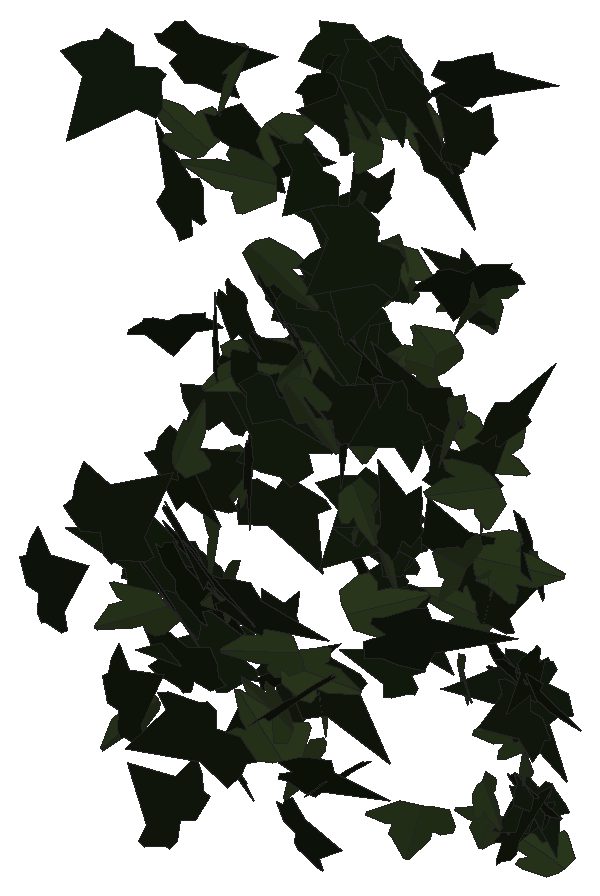
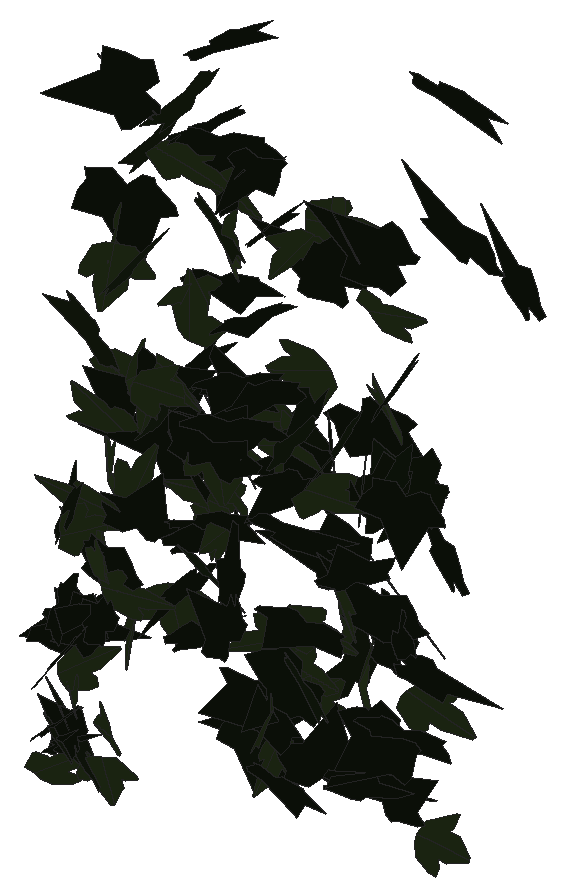
# SketchUp Ruby script. Lengths in inches.
U = 1.inch
M = Sketchup.active_model
def pt(a) = Geom::Point3d.new(a.map { |v| v * U })
def face(e, loops, mat)
  f = e.add_face(loops[0].map { |a| pt(a) })
  loops[1..].each { |l| e.add_face(l.map { |a| pt(a) }).erase! }
  f.material = f.back_material = mat if mat
  f
end
# faces: each face lists its corners as indices into pts; further lists are holes
def faces(e, pts, list, mat = nil) = list.each { |f| face(e, (f[0].is_a?(Array) ? f : [f]).map { |l| l.map { |i| pts[i] } }, mat) }
# xy, xz, yz: faces in a plane at the given z, y or x. An outline is a flat list of corners, or four numbers for a rectangle; further outlines are holes
def ring(l) = l.size == 4 ? [[l[0], l[1]], [l[2], l[1]], [l[2], l[3]], [l[0], l[3]]] : l.each_slice(2).to_a
def flat(e, list, mat, &to3) = list.each { |f| face(e, (f[0].is_a?(Array) ? f : [f]).map { |l| ring(l).map { |u, v| to3.(u, v) } }, mat) }
def xy(e, z, list, mat = nil) = flat(e, list, mat) { |x, y| [x, y, z] }
def xz(e, y, list, mat = nil) = flat(e, list, mat) { |x, z| [x, y, z] }
def yz(e, x, list, mat = nil) = flat(e, list, mat) { |y, z| [x, y, z] }
def lines(e, pts, list) = list.each { |a, b| e.add_line(pt(pts[a]), pt(pts[b])) }
# prism: a flat outline (further loops are holes) pulled along v
def prism(e, loops, v, mat = nil)
  f = face(e, loops, mat); d = Geom::Vector3d.new(v.map { |x| x * U })
  f.pushpull(f.normal.samedirection?(d) ? d.length : -d.length)
end
def box(e, o, s, mat = nil) = prism(e, [[o, [o[0] + s[0], o[1], o[2]], [o[0] + s[0], o[1] + s[1], o[2]], [o[0], o[1] + s[1], o[2]]]], [0, 0, s[2]], mat)
def at(x, y, z, deg = 0) = Geom::Transformation.translation(pt([x, y, z])) * Geom::Transformation.rotation(ORIGIN, Z_AXIS, deg.degrees)
def axes(o, x, y, z) = Geom::Transformation.new([*x, 0, *y, 0, *z, 0, *pt(o).to_a, 1])
def part(name) = M.definitions.add(name)
# library, detail: a bought-in or finely detailed component or shape, given as its bounding box
def library(name, o, s) = part(name).tap { |d| box(d.entities, o, s) }
def detail(e, o, s) = box(e.add_group.entities, o, s)
def put(e, d, t, mat = nil) = e.add_instance(d, t).tap { |i| i.material = mat if mat }
def group(e, t, mat = nil) = e.add_group.tap { |g| g.transformation = t; g.material = mat if mat }.entities
root = M.entities
M.materials.add("1026 AP 7946 SUNNY SIDE UP").color = [254, 231, 186]
M.materials.add("efeu1").color = [18, 25, 13]
M.materials.add("efeu2").color = [43, 57, 29]
c1 = part("ivyleaf_9")
p = [[1.54,2.16,1.25],[1.36,2.04,1.19],[-0.21,0.99,0.68],[-0.71,1.11,0.82],[-0.85,0.86,0.67],[-0.8,0.17,0.21],
  [-0.9,-0.01,0.1],[-0.67,-0.16,-0.02],[-0.08,-0.08,-0.05],[-0.03,-0.6,-0.4],[0.65,-0.88,-0.66],[0.83,-0.6,-0.49],
  [1.29,-0.42,-0.43],[1.8125,-0.07,-0.26],[1.21,0.44,0.15]]
faces(c1.entities,p,[[0,1,2,3,4,5,6,7,8,9,10,11,12,13,14]],"efeu1")
c2 = part("ivyleaf_10")
p = [[0,0.5,-0.03],[-0.0625,2.02,-0.43],[-0.19,2.01,-0.46],[-0.54,1.05,-0.29],[-0.52,0.625,-0.18],[-0.83,0.76,-0.28],
  [-1.16,0.64,-0.33],[-1.15,0.33,-0.24],[-0.77,-0.39,0.02],[-0.3,-0.51,0.16],[0.04,-0.48,0.23],[-0.02,2.01,-0.4375],
  [-0.06,2.01,-0.43],[0.04,-0.49,0.23],[0.67,-0.49,0.14],[1.38,0.36,-0.2],[1.375,0.51,-0.24],[0.81,0.65,-0.19],
  [0.62,0.59,-0.15],[0.6,1.09,-0.28],[0.5,1.23,-0.31]]
faces(c2.entities,p,[[0,1,2,3,4,5,6,7,8,9,10],[11,12,0,13,14,15,16,17,18,19,20]],"efeu2")
put(root,c1,axes([134.92,203.27,273.71],[-0.05413,0.16337,0.43525],[0.20214,-0.40179,0.16888],[0.68156,0.13214,-0.01552]),"1026 AP 7946 SUNNY SIDE UP")
put(root,c1,axes([135.52,203.9,274.61],[-0.26884,0.25267,0.37218],[0.36214,-0.27742,0.31179],[0.58893,0.28592,-0.02182]),"1026 AP 7946 SUNNY SIDE UP")
put(root,c1,axes([136.9,204.57,271.65],[0.09194,0.02172,-0.4349],[-0.55596,-0.23128,-0.06404],[-0.36463,0.35811,-0.01201]),"1026 AP 7946 SUNNY SIDE UP")
put(root,c1,axes([135.65,205.37,269.47],[-0.1744,0.29145,0.36963],[-0.22633,0.32707,-0.31911],[-0.68858,-0.18132,0.01127]),"1026 AP 7946 SUNNY SIDE UP")
put(root,c1,axes([134.24,205.87,270.5],[-0.06985,0.19411,0.41803],[0.15581,-0.39238,0.20281],[0.68832,0.10852,-0.00348]),"1026 AP 7946 SUNNY SIDE UP")
put(root,c1,axes([137.46,205.68,271.87],[-0.04372,0.43292,-0.00427],[-0.01045,-0.00704,-0.44689],[-0.68072,-0.0277,0.00713]),"1026 AP 7946 SUNNY SIDE UP")
put(root,c1,axes([137.85,206.92,278.61],[-0.34789,-0.28295,0.25193],[-0.17642,-0.22276,-0.36899],[0.5627,-0.24478,0.04006]),"1026 AP 7946 SUNNY SIDE UP")
put(root,c1,axes([134.03,206.58,272.41],[0.5694,-0.19458,-0.13462],[-0.20254,0.03327,-0.42216],[0.30674,0.38316,-0.02887]),"1026 AP 7946 SUNNY SIDE UP")
put(root,c1,axes([134.3,207.28,272.5],[0.03012,-0.22503,0.3574],[0.10519,-0.34233,-0.23371],[0.64336,0.06651,0.02148]),"1026 AP 7946 SUNNY SIDE UP")
put(root,c1,axes([133.29,207.28,279.61],[-0.654,-0.06761,-0.09489],[0.15218,-0.02632,-0.43224],[0.09459,-0.4251,0.0393]),"1026 AP 7946 SUNNY SIDE UP")
put(root,c1,axes([134.24,207.27,272.38],[0.38274,-0.24837,0.19976],[0.18036,-0.16027,-0.35816],[0.46293,0.26779,-0.02561]),"1026 AP 7946 SUNNY SIDE UP")
put(root,c1,axes([134.77,207.46,269.28],[0.39766,-0.22936,-0.16384],[0.21644,-0.08219,0.35],[-0.38043,-0.2865,0.02787]),"1026 AP 7946 SUNNY SIDE UP")
put(root,c2,axes([134.14,207.39,273.78],[0.43785,-0.28476,0.01508],[0.01326,0.03093,0.4095],[-0.44829,-0.27722,0.02685]),"1026 AP 7946 SUNNY SIDE UP")
put(root,c2,axes([138.17,207.52,269.47],[-0.41659,-0.25148,0.06461],[-0.04462,-0.06305,-0.37575],[0.40564,-0.2652,0.02502]),"1026 AP 7946 SUNNY SIDE UP")
put(root,c1,axes([137.77,207.4,272.21],[0.2143,0.23659,-0.36215],[0.18766,0.33435,0.28038],[0.64114,-0.17694,0.03898]),"1026 AP 7946 SUNNY SIDE UP")
put(root,c1,axes([134.61,207.81,271.45],[0.33293,-0.06746,0.30215],[0.41934,-0.12513,-0.22842],[0.22055,0.33974,-0.0218]),"1026 AP 7946 SUNNY SIDE UP")
put(root,c1,axes([134.58,208.25,273.58],[-0.09542,-0.00754,-0.37178],[0.50938,-0.16245,-0.05358],[-0.25019,-0.32787,0.03271]),"1026 AP 7946 SUNNY SIDE UP")
put(root,c1,axes([135.39,208.3125,267.85],[0.06947,-0.04418,0.33011],[0.23093,-0.28569,-0.06306],[0.4536,0.15221,-0.01845]),"1026 AP 7946 SUNNY SIDE UP")
put(root,c2,axes([135.08,208.1875,269.17],[0.45185,0.1023,0.19594],[-0.30209,-0.02141,0.31172],[0.15334,-0.34362,0.03672]),"1026 AP 7946 SUNNY SIDE UP")
put(root,c2,axes([136.7,208.1,271.94],[0.17937,0.03263,-0.3553],[0.44402,0.2019,0.11702],[0.31604,-0.30219,0.03724]),"1026 AP 7946 SUNNY SIDE UP")
put(root,c2,axes([135.18,208.1875,269.625],[-0.08054,0.00433,-0.36622],[-0.40282,0.24861,0.0426],[0.38765,0.25924,-0.03182]),"1026 AP 7946 SUNNY SIDE UP")
put(root,c2,axes([135.06,208.43,270.54],[-0.16869,-0.007,0.32375],[-0.44249,-0.14593,-0.10315],[0.2204,-0.29833,0.0407]),"1026 AP 7946 SUNNY SIDE UP")
put(root,c2,axes([133.9375,208.6875,271.12],[-0.01153,-0.01036,-0.38201],[-0.08514,-0.36682,0.00952],[-0.57695,0.05434,0.00623]),"1026 AP 7946 SUNNY SIDE UP")
put(root,c1,axes([133.05,208.62,270.87],[0.10197,-0.07645,0.37883],[0.24558,-0.33437,-0.10182],[0.53784,0.16717,-0.02533]),"1026 AP 7946 SUNNY SIDE UP")
put(root,c1,axes([135.29,208.4375,268.71],[0.36077,0.01767,0.23075],[0.35276,-0.00325,-0.2366],[-0.0163,0.32056,-0.01324]),"1026 AP 7946 SUNNY SIDE UP")
put(root,c2,axes([132.55,208.7,270.21],[-0.24903,-0.12302,0.29395],[-0.3272,-0.1969,-0.20709],[0.36421,-0.26101,0.01494]),"1026 AP 7946 SUNNY SIDE UP")
put(root,c2,axes([134.39,208.67,277.62],[0.03862,-0.03624,-0.37202],[-0.56524,-0.05077,-0.02025],[-0.07622,0.35817,-0.03835]),"1026 AP 7946 SUNNY SIDE UP")
put(root,c2,axes([135.25,208.55,270.27],[0.09481,0.10228,0.31314],[0.27804,0.24672,-0.12045],[-0.41967,0.18656,-0.00905]),"1026 AP 7946 SUNNY SIDE UP")
put(root,c1,axes([135.66,208.8125,274.25],[-0.17911,0.15665,0.31447],[0.32966,-0.22164,0.19706],[0.42548,0.23767,-0.0203]),"1026 AP 7946 SUNNY SIDE UP")
put(root,c1,axes([134.22,208.9,268.5],[0.39518,0.10777,0.2429],[-0.3634,-0.05377,0.27951],[0.18275,-0.33997,0.03055]),"1026 AP 7946 SUNNY SIDE UP")
put(root,c1,axes([136.55,209.22,274.51],[0.14068,-0.22493,-0.35866],[0.25272,-0.30806,0.24669],[-0.59891,-0.18282,0.01985]),"1026 AP 7946 SUNNY SIDE UP")
put(root,c2,axes([138.16,208.91,273.99],[0.32589,-0.07536,-0.28685],[-0.43216,0.05077,-0.22496],[0.13556,0.34303,-0.02758]),"1026 AP 7946 SUNNY SIDE UP")
put(root,c2,axes([134.89,209.01,274.25],[-0.29978,0.12286,-0.30645],[0.34398,-0.20522,-0.23242],[-0.37257,-0.28833,0.03199]),"1026 AP 7946 SUNNY SIDE UP")
put(root,c2,axes([132.01,209.16,268.27],[-0.03962,-0.21687,0.31043],[-0.00532,-0.30311,-0.22588],[0.58531,-0.01744,0.01896]),"1026 AP 7946 SUNNY SIDE UP")
put(root,c1,axes([132.52,208.95,270.91],[-0.24743,-0.11187,-0.32004],[-0.45117,-0.12255,0.19488],[-0.25501,0.32536,-0.03424]),"1026 AP 7946 SUNNY SIDE UP")
put(root,c1,axes([135.7,208.78,268.63],[0.02821,0.30252,0.03014],[0.00077,0.02755,-0.31204],[-0.47765,0.01791,0.00127]),"1026 AP 7946 SUNNY SIDE UP")
put(root,c2,axes([135.1,208.85,268.62],[-0.05097,-0.28898,-0.25893],[0.13822,0.23823,-0.29438],[0.5844,-0.08155,0.04704]),"1026 AP 7946 SUNNY SIDE UP")
put(root,c2,axes([135.6875,209.21,272.87],[0.27893,-0.04602,0.26804],[0.37245,-0.11186,-0.18722],[0.185,0.29459,-0.02721]),"1026 AP 7946 SUNNY SIDE UP")
put(root,c1,axes([134.9,209.42,277.6],[-0.15127,-0.23839,0.23479],[-0.11584,-0.21732,-0.26591],[0.507,-0.12078,0.0093]),"1026 AP 7946 SUNNY SIDE UP")
put(root,c2,axes([137.43,209.4,272.29],[-0.06813,-0.23645,-0.33017],[-0.13001,-0.30865,0.24533],[-0.61088,0.09206,-0.01539]),"1026 AP 7946 SUNNY SIDE UP")
put(root,c1,axes([137.77,209.05,277.15],[0.20154,0.36464,-0.14214],[-0.04982,-0.1372,-0.3987],[-0.61216,0.13122,-0.01435]),"1026 AP 7946 SUNNY SIDE UP")
put(root,c1,axes([135.75,209.34,276.47],[-0.41766,-0.24427,-0.10368],[0.14444,0.04632,-0.37044],[0.38861,-0.27975,0.02626]),"1026 AP 7946 SUNNY SIDE UP")
put(root,c1,axes([135.41,209.39,274.1875],[-0.20732,0.03604,-0.39047],[0.53335,-0.17155,-0.13929],[-0.27264,-0.363,0.02444]),"1026 AP 7946 SUNNY SIDE UP")
put(root,c1,axes([136.73,208.91,272.74],[0.00295,0.12141,0.40988],[-0.15199,0.38641,-0.11895],[-0.63512,-0.0919,0.03037]),"1026 AP 7946 SUNNY SIDE UP")
put(root,c1,axes([134.67,208.92,269.92],[0.2829,0.29186,0.21303],[0.19633,0.16369,-0.35179],[-0.52545,0.2183,-0.01675]),"1026 AP 7946 SUNNY SIDE UP")
put(root,c2,axes([135.52,209.49,277.23],[0.21093,-0.27501,0.26184],[0.21687,-0.21649,-0.31565],[0.54922,0.19111,0.02408]),"1026 AP 7946 SUNNY SIDE UP")
put(root,c2,axes([135.98,209.37,272.23],[-0.26746,0.17063,-0.20001],[0.15733,-0.17207,-0.24588],[-0.37598,-0.19338,0.03939]),"1026 AP 7946 SUNNY SIDE UP")
put(root,c1,axes([136.42,209.47,270.21],[-0.13996,0.02824,0.28755],[-0.36696,-0.16968,-0.06001],[0.24436,-0.23864,0.07457]),"1026 AP 7946 SUNNY SIDE UP")
put(root,c2,axes([137.16,209.63,274.41],[0.07735,-0.10176,0.39822],[0.2715,-0.34649,-0.11846],[0.56783,0.17953,0.00239]),"1026 AP 7946 SUNNY SIDE UP")
put(root,c1,axes([134.88,209.4375,269.67],[-0.08907,-0.06535,-0.41877],[0.60162,0.14217,-0.07771],[0.23751,-0.38462,0.03981]),"1026 AP 7946 SUNNY SIDE UP")
put(root,c2,axes([137.73,209.19,276.67],[-0.01977,-0.19648,-0.3041],[0.01433,0.29398,-0.20103],[0.55593,-0.01457,-0.00563]),"1026 AP 7946 SUNNY SIDE UP")
put(root,c1,axes([137.48,209.25,273.6875],[-0.14343,-0.06397,0.34863],[0.46595,0.16457,0.11517],[-0.27708,0.30985,0.01321]),"1026 AP 7946 SUNNY SIDE UP")
put(root,c1,axes([132.23,209.56,271.97],[0.07702,-0.08004,-0.33046],[0.51913,0.00855,0.04986],[-0.00533,-0.32393,0.08095]),"1026 AP 7946 SUNNY SIDE UP")
put(root,c1,axes([135.88,209.72,272.52],[-0.48893,-0.25258,0.11222],[-0.0935,-0.101,-0.41128],[0.42321,-0.31411,0.03878]),"1026 AP 7946 SUNNY SIDE UP")
put(root,c1,axes([132.64,209.43,268.85],[0.12631,-0.0451,0.33373],[-0.38105,0.21621,0.09411],[-0.34598,-0.25459,0.01819]),"1026 AP 7946 SUNNY SIDE UP")
put(root,c1,axes([137.67,209.27,279.02],[-0.03263,0.1638,0.32255],[-0.22761,0.28117,-0.16026],[-0.50544,-0.13719,0.05134]),"1026 AP 7946 SUNNY SIDE UP")
put(root,c2,axes([132.76,209.76,270.95],[0.01789,-0.08048,0.40028],[0.36605,-0.31399,-0.07577],[0.50613,0.22993,0.04065]),"1026 AP 7946 SUNNY SIDE UP")
put(root,c1,axes([136.12,209.58,279.48],[0.32383,-0.37927,-0.0374],[-0.01997,0.03196,-0.4444],[0.59845,0.2063,0.00541]),"1026 AP 7946 SUNNY SIDE UP")
put(root,c1,axes([136.27,209.38,271.29],[0.22801,-0.24677,-0.29964],[-0.17693,0.26808,-0.29195],[0.57132,0.18151,0.02917]),"1026 AP 7946 SUNNY SIDE UP")
put(root,c1,axes([136.25,209.48,271.73],[-0.36435,0.19664,0.01676],[-0.04034,-0.00688,-0.31231],[-0.30748,-0.23211,0.02112]),"1026 AP 7946 SUNNY SIDE UP")
put(root,c1,axes([136.28,209.66,271.98],[-0.17344,0.02993,0.28901],[-0.39175,-0.15131,-0.08523],[0.20759,-0.26054,0.08063]),"1026 AP 7946 SUNNY SIDE UP")
put(root,c1,axes([132.48,209.52,271.86],[-0.13447,0.08732,0.38273],[0.48792,-0.20486,0.12215],[0.34803,0.32094,-0.02338]),"1026 AP 7946 SUNNY SIDE UP")
put(root,c2,axes([134.74,209.58,269.59],[-0.16201,0.351,-0.14854],[0.04153,-0.14448,-0.37741],[-0.59642,-0.10541,0.01407]),"1026 AP 7946 SUNNY SIDE UP")
put(root,c1,axes([133.36,209.58,277.35],[0.12069,0.00153,0.41724],[0.51844,-0.23962,-0.06484],[0.36983,0.33541,-0.04526]),"1026 AP 7946 SUNNY SIDE UP")
put(root,c1,axes([136.75,209.65,278.51],[0.23791,-0.31756,0.00658],[-0.01356,-0.01317,-0.36219],[0.49931,0.15095,-0.01297]),"1026 AP 7946 SUNNY SIDE UP")
put(root,c1,axes([138.13,209.33,274.69],[-0.23263,0.36839,0.0038],[0.01393,0.00184,0.40888],[0.5791,0.14794,-0.00831]),"1026 AP 7946 SUNNY SIDE UP")
put(root,c1,axes([134.25,209.3,270.17],[-0.03252,0.20273,0.28469],[-0.09734,0.26892,-0.20731],[-0.52857,-0.062,0.02066]),"1026 AP 7946 SUNNY SIDE UP")
put(root,c1,axes([136.72,209.5,274.32],[0.14268,-0.01682,0.3496],[-0.40018,0.22949,0.08314],[-0.35418,-0.26607,0.04689]),"1026 AP 7946 SUNNY SIDE UP")
put(root,c1,axes([138.21,209.85,270.08],[0.14761,-0.23368,-0.25507],[0.1625,-0.22371,0.25797],[-0.50848,-0.13933,0.00839]),"1026 AP 7946 SUNNY SIDE UP")
put(root,c2,axes([133.77,209.64,275.76],[-0.29718,0.0644,-0.32208],[0.44011,-0.14212,-0.20506],[-0.24247,-0.33689,0.02255]),"1026 AP 7946 SUNNY SIDE UP")
put(root,c2,axes([134.25,209.69,274.37],[0.57149,-0.06577,0.13578],[0.19152,-0.0649,-0.37868],[0.13119,0.38126,-0.03867]),"1026 AP 7946 SUNNY SIDE UP")
put(root,c2,axes([135.72,209.34,272.28],[0.08421,0.00414,0.35279],[-0.16452,0.33021,0.01468],[-0.51273,-0.10528,0.05323]),"1026 AP 7946 SUNNY SIDE UP")
put(root,c1,axes([135.8,209.36,277.37],[-0.00072,0.21466,0.28259],[-0.11444,0.26697,-0.21475],[-0.53406,-0.05749,0.04564]),"1026 AP 7946 SUNNY SIDE UP")
put(root,c1,axes([133.8,209.55,275.41],[0.39384,-0.14466,-0.18501],[-0.24822,0.08406,-0.29744],[0.26295,0.29602,-0.00367]),"1026 AP 7946 SUNNY SIDE UP")
put(root,c1,axes([135.13,209.63,273.66],[-0.08255,0.24678,0.24551],[0.0955,-0.22915,0.25843],[0.52936,0.07983,-0.00834]),"1026 AP 7946 SUNNY SIDE UP")
put(root,c1,axes([133.17,209.6,274.91],[0.28767,-0.23408,-0.16684],[-0.17779,0.11519,-0.30495],[0.40945,0.21448,-0.0152]),"1026 AP 7946 SUNNY SIDE UP")
put(root,c2,axes([134.375,209.42,274.1875],[0.09462,-0.13726,0.3159],[-0.05938,0.30757,0.15089],[-0.52605,-0.05941,0.03979]),"1026 AP 7946 SUNNY SIDE UP")
put(root,c1,axes([133.5625,209.64,274.14],[0.0721,-0.05905,-0.39254],[0.49322,0.2283,0.00378],[0.35169,-0.30808,0.07518]),"1026 AP 7946 SUNNY SIDE UP")
put(root,c2,axes([133.34,209.67,272.27],[0.32371,-0.27325,-0.1215],[-0.1005,0.09753,-0.3518],[0.45607,0.21544,0.00871]),"1026 AP 7946 SUNNY SIDE UP")
put(root,c2,axes([135.61,209.59,278.27],[0.11016,-0.08691,-0.33732],[-0.42143,0.18947,-0.10995],[0.32458,0.2755,-0.02827]),"1026 AP 7946 SUNNY SIDE UP")
put(root,c1,axes([136.3,209.95,274.29],[0.09247,-0.38334,0.16065],[0.02574,-0.15743,-0.40039],[0.65152,0.06063,-0.00698]),"1026 AP 7946 SUNNY SIDE UP")
put(root,c1,axes([133.01,209.52,273.8125],[-0.02278,-0.09547,0.33235],[0.07623,0.31949,0.10135],[-0.52432,0.0506,0.00029]),"1026 AP 7946 SUNNY SIDE UP")
put(root,c2,axes([133.14,209.84,278.57],[0.32392,-0.31036,0.12859],[0.08019,-0.11782,-0.38381],[0.52091,0.21114,-0.02088]),"1026 AP 7946 SUNNY SIDE UP")
put(root,c1,axes([135.14,209.96,278.26],[-0.11788,-0.02653,0.35837],[-0.32714,-0.2824,-0.07],[0.44064,-0.21675,0.0439]),"1026 AP 7946 SUNNY SIDE UP")
put(root,c1,axes([133.1,209.86,269.15],[-0.38956,-0.00795,0.25357],[-0.3766,-0.07372,-0.25119],[0.0904,-0.34139,0.04625]),"1026 AP 7946 SUNNY SIDE UP")
put(root,c1,axes([131.99,209.8,270.39],[-0.28027,-0.2035,-0.25405],[0.32672,0.13914,-0.27348],[0.38026,-0.26954,0.04773]),"1026 AP 7946 SUNNY SIDE UP")
put(root,c2,axes([135.53,209.76,273.81],[-0.36728,-0.29942,0.02744],[0.00324,-0.03747,-0.39062],[0.47291,-0.23229,0.02399]),"1026 AP 7946 SUNNY SIDE UP")
put(root,c2,axes([133.5,209.91,273.93],[0.27848,0.1196,-0.32514],[-0.35777,-0.22197,-0.21902],[-0.39332,0.28658,-0.03098]),"1026 AP 7946 SUNNY SIDE UP")
put(root,c2,axes([135.94,209.8125,276.45],[0.25895,0.25587,-0.12449],[-0.07331,-0.11507,-0.31337],[-0.43986,0.16981,-0.02106]),"1026 AP 7946 SUNNY SIDE UP")
put(root,c1,axes([132.1,209.62,274.17],[0.23702,0.28887,-0.07523],[-0.04397,-0.06961,-0.33599],[-0.46708,0.15314,-0.00655]),"1026 AP 7946 SUNNY SIDE UP")
put(root,c2,axes([132.52,209.71,277.16],[0.25533,0.08308,0.28855],[-0.45249,-0.00677,0.17419],[0.07509,-0.32328,0.06849]),"1026 AP 7946 SUNNY SIDE UP")
put(root,c1,axes([134,209.7,273.84],[-0.01812,-0.21628,-0.29974],[0.08749,0.28536,-0.22006],[0.56173,-0.05142,0.02461]),"1026 AP 7946 SUNNY SIDE UP")
put(root,c2,axes([134.01,209.62,277.81],[0.1383,0.26208,0.20518],[0.08066,0.19116,-0.28349],[-0.50984,0.10134,0.01081]),"1026 AP 7946 SUNNY SIDE UP")
put(root,c1,axes([135.57,209.92,279.4],[0.00623,-0.37484,-0.05757],[0.0026,0.05378,-0.38585],[0.59542,0.00369,0.00229]),"1026 AP 7946 SUNNY SIDE UP")
put(root,c2,axes([137.37,209.9375,268.51],[0.15333,-0.02495,0.28736],[0.37186,-0.15114,-0.09993],[0.23627,0.25406,-0.0292]),"1026 AP 7946 SUNNY SIDE UP")
put(root,c1,axes([134.35,209.77,272.875],[-0.54477,-0.13175,-0.17402],[-0.26669,-0.02517,0.38015],[-0.20424,0.38429,-0.03224]),"1026 AP 7946 SUNNY SIDE UP")
put(root,c1,axes([135.07,210,271.78],[0.071,0.15827,0.36968],[-0.19651,-0.33563,0.16716],[0.58319,-0.13236,0.01132]),"1026 AP 7946 SUNNY SIDE UP")
put(root,c1,axes([132.24,209.74,270.16],[0.64019,-0.02729,-0.0229],[-0.03863,-0.03807,-0.41862],[0.03941,0.40596,-0.03839]),"1026 AP 7946 SUNNY SIDE UP")
put(root,c1,axes([136.9,209.89,272.17],[0.33013,0.00189,0.21581],[-0.32605,0.044,0.21396],[-0.04679,-0.2933,0.03174]),"1026 AP 7946 SUNNY SIDE UP")
put(root,c2,axes([137.42,209.82,276.45],[-0.30189,-0.32511,-0.10117],[0.1093,0.07065,-0.38782],[0.52187,-0.20287,0.0227]),"1026 AP 7946 SUNNY SIDE UP")
put(root,c2,axes([137.28,210.05,273],[-0.07978,0.0727,0.33031],[0.3524,-0.22915,0.08884],[0.37737,0.22936,-0.01313]),"1026 AP 7946 SUNNY SIDE UP")
put(root,c1,axes([132.28,209.83,275.85],[-0.12932,-0.31392,0.25376],[0.11497,0.23723,0.33559],[-0.61857,0.10972,0.00932]),"1026 AP 7946 SUNNY SIDE UP")
put(root,c1,axes([134.64,209.98,275.32],[-0.22282,-0.33234,-0.19445],[0.1438,0.1639,-0.3708],[0.58201,-0.16773,0.01717]),"1026 AP 7946 SUNNY SIDE UP")
put(root,c2,axes([137.55,209.92,272.21],[0.08373,-0.10106,-0.37871],[0.58225,-0.07229,0.07542],[-0.13897,-0.36376,0.08784]),"1026 AP 7946 SUNNY SIDE UP")
put(root,c1,axes([137.77,209.9,267.89],[-0.02942,0.33581,0.26334],[0.02981,-0.25303,0.34498],[0.66112,0.02635,-0.00384]),"1026 AP 7946 SUNNY SIDE UP")
put(root,c1,axes([137.2,210.09,276.2],[0.09128,-0.36434,-0.00821],[0.02153,-0.00379,0.37982],[-0.57256,-0.05823,0.01297]),"1026 AP 7946 SUNNY SIDE UP")
put(root,c2,axes([137.09,209.82,270.32],[-0.22003,0.23053,0.09356],[-0.11851,0.05819,-0.27545],[-0.37035,-0.15558,0.03256]),"1026 AP 7946 SUNNY SIDE UP")
put(root,c1,axes([134.75,209.7,278.97],[0.00251,-0.05464,-0.35124],[-0.18102,0.32103,-0.05172],[0.51137,0.11391,-0.01659]),"1026 AP 7946 SUNNY SIDE UP")
put(root,c2,axes([136.17,209.98,278.68],[0.34538,-0.032,-0.32416],[-0.4969,-0.01301,-0.2261],[0.01197,0.38337,-0.03247]),"1026 AP 7946 SUNNY SIDE UP")
put(root,c2,axes([137.88,210.1875,269.53],[-0.01752,0.10103,0.36719],[-0.0278,-0.35576,0.1014],[0.581,-0.01397,0.01593]),"1026 AP 7946 SUNNY SIDE UP")
put(root,c1,axes([135.02,210.15,271.05],[0.14877,-0.15909,0.32771],[0.19125,-0.29584,-0.19088],[0.52689,0.1523,-0.02325]),"1026 AP 7946 SUNNY SIDE UP")
put(root,c2,axes([136.43,209.87,274.89],[-0.11471,0.08449,0.30389],[-0.46674,0.05551,-0.09183],[-0.11935,-0.29828,0.06705]),"1026 AP 7946 SUNNY SIDE UP")
put(root,c1,axes([132.11,209.91,278.26],[0.51084,0.04841,-0.21588],[0.25796,0.19038,0.30803],[0.21934,-0.33664,0.14052]),"1026 AP 7946 SUNNY SIDE UP")
put(root,c1,axes([135.1875,210.11,279.36],[-0.37542,-0.30031,-0.16578],[0.19328,0.10511,-0.39353],[0.4983,-0.26703,0.02775]),"1026 AP 7946 SUNNY SIDE UP")
put(root,c1,axes([138.08,210.23,270.59],[-0.06238,-0.00403,-0.36587],[0.33828,-0.28458,-0.0231],[-0.44431,-0.2161,0.03378]),"1026 AP 7946 SUNNY SIDE UP")
put(root,c2,axes([136.67,209.95,274.49],[-0.36105,0.20825,0.02633],[-0.04999,0.00115,-0.31865],[-0.32588,-0.2309,0.01971]),"1026 AP 7946 SUNNY SIDE UP")
put(root,c1,axes([135.41,210.05,273.88],[0.42667,-0.10805,0.27527],[-0.35061,0.15515,0.29813],[-0.28858,-0.34826,0.04477]),"1026 AP 7946 SUNNY SIDE UP")
put(root,c1,axes([133.7,210.23,274.78],[0.12133,-0.32012,0.17313],[0.04613,-0.16759,-0.34007],[0.56797,0.082,-0.00936]),"1026 AP 7946 SUNNY SIDE UP")
put(root,c2,axes([135.76,210.03,275.97],[-0.549,0.1673,0.07803],[0.12853,-0.00186,0.39739],[0.2579,0.35707,-0.03194]),"1026 AP 7946 SUNNY SIDE UP")
put(root,c2,axes([137.32,210.2,271.42],[0.02886,-0.24226,-0.19628],[0.05131,-0.18688,0.24875],[-0.48056,-0.0345,0.01477]),"1026 AP 7946 SUNNY SIDE UP")
put(root,c2,axes([137.42,210.06,268.01],[-0.38236,-0.07279,0.07666],[-0.10159,-0.04407,-0.2607],[0.12894,-0.25058,0.02194]),"1026 AP 7946 SUNNY SIDE UP")
put(root,c1,axes([134.53,210.26,276.66],[-0.13471,-0.3659,-0.00109],[0.01271,-0.00294,-0.38706],[0.5752,-0.08563,0.0083]),"1026 AP 7946 SUNNY SIDE UP")
put(root,c1,axes([133.6,210.11,271.78],[-0.18896,-0.17599,-0.29203],[0.34864,0.18163,-0.2127],[0.39027,-0.24747,0.04861]),"1026 AP 7946 SUNNY SIDE UP")
put(root,c1,axes([137.11,210.14,271.32],[-0.05712,0.07964,0.35019],[0.33761,-0.26382,0.08589],[0.43201,0.2167,-0.02082]),"1026 AP 7946 SUNNY SIDE UP")
put(root,c1,axes([138.12,210.3125,270.27],[-0.11019,-0.14586,-0.34272],[-0.15108,-0.31843,0.16322],[-0.54959,0.11678,0.02385]),"1026 AP 7946 SUNNY SIDE UP")
put(root,c2,axes([137.28,210,273.8125],[0.46466,-0.01979,-0.19768],[0.30274,0.04829,0.3008],[0.01555,-0.34896,0.05075]),"1026 AP 7946 SUNNY SIDE UP")
put(root,c1,axes([138.09,210.29,268.26],[-0.18386,-0.12655,0.1928],[-0.17077,-0.15421,-0.17755],[0.31256,-0.1587,0.0164]),"1026 AP 7946 SUNNY SIDE UP")
put(root,c1,axes([134.88,210.26,274.75],[-0.38983,-0.30296,-0.14104],[0.17974,0.08042,-0.40116],[0.4897,-0.27069,0.03496]),"1026 AP 7946 SUNNY SIDE UP")
put(root,c2,axes([137.8,210.34,271.95],[0.01937,0.00303,-0.34589],[-0.27738,-0.28583,-0.01099],[-0.44925,0.17661,-0.00813]),"1026 AP 7946 SUNNY SIDE UP")
put(root,c2,axes([138.38,210.18,267.66],[0.17277,0.16715,0.2099],[-0.20237,-0.15742,0.20458],[0.36028,-0.16858,0.01426]),"1026 AP 7946 SUNNY SIDE UP")
put(root,c1,axes([132.76,209.97,272.74],[-0.32523,-0.08749,0.2587],[0.33594,0.13579,0.23037],[-0.25019,0.29606,-0.02696]),"1026 AP 7946 SUNNY SIDE UP")
put(root,c2,axes([137.8,210.25,269.05],[-0.0727,0.05434,0.27934],[0.32624,-0.17448,0.07153],[0.28678,0.21226,-0.01055]),"1026 AP 7946 SUNNY SIDE UP")
put(root,c2,axes([137.1,210.15,271.09],[0.06572,0.05722,0.32237],[-0.46562,-0.10743,0.06042],[0.18138,-0.29652,0.0383]),"1026 AP 7946 SUNNY SIDE UP")
put(root,c1,axes([134.72,210.18,275.51],[-0.12086,-0.31934,-0.18736],[0.10804,0.16816,-0.33649],[0.56624,-0.10025,0.02421]),"1026 AP 7946 SUNNY SIDE UP")
put(root,c1,axes([134,210.25,269.08],[-0.44466,-0.08119,-0.17266],[0.26788,0.00824,-0.30102],[0.11665,-0.32839,0.0331]),"1026 AP 7946 SUNNY SIDE UP")
put(root,c1,axes([138.1,210.25,268.61],[0.04674,-0.2849,-0.00404],[-0.00325,0.0021,-0.29507],[0.44798,0.02974,-0.00172]),"1026 AP 7946 SUNNY SIDE UP")
put(root,c1,axes([137.63,210.1,270.37],[0.47079,-0.06913,0.09864],[0.13506,-0.05317,-0.31526],[0.12818,0.30994,-0.03012]),"1026 AP 7946 SUNNY SIDE UP")
put(root,c1,axes([137.79,210.25,268.49],[0.28394,-0.05393,-0.20538],[0.31773,-0.00659,0.19065],[-0.06479,-0.26867,0.03492]),"1026 AP 7946 SUNNY SIDE UP")
put(root,c1,axes([137.875,210.14,270.02],[0.26373,-0.30547,-0.17446],[-0.1487,0.13913,-0.35789],[0.52731,0.19201,-0.01367]),"1026 AP 7946 SUNNY SIDE UP")
put(root,c1,axes([136.83,209.92,279.48],[0.3127,0.11911,0.32754],[0.46406,0.11992,-0.23626],[-0.2619,0.35472,-0.02756]),"1026 AP 7946 SUNNY SIDE UP")
put(root,c2,axes([136.32,210.38,274.9],[-0.11395,-0.11911,0.31643],[-0.14554,-0.29519,-0.14184],[0.49818,-0.11348,0.03094]),"1026 AP 7946 SUNNY SIDE UP")
put(root,c1,axes([137.21,210.31,270.51],[0.13006,-0.12611,0.23726],[0.15989,-0.20805,-0.15572],[0.38172,0.13011,-0.01561]),"1026 AP 7946 SUNNY SIDE UP")
put(root,c1,axes([137.82,210.45,272.13],[-0.04032,-0.09536,0.38473],[-0.04807,-0.37314,-0.10235],[0.60497,-0.03601,0.01751]),"1026 AP 7946 SUNNY SIDE UP")
put(root,c1,axes([138.2,210.24,268.44],[-0.33191,0.10413,-0.1481],[0.18128,-0.09062,-0.24154],[-0.21323,-0.23913,0.02518]),"1026 AP 7946 SUNNY SIDE UP")
